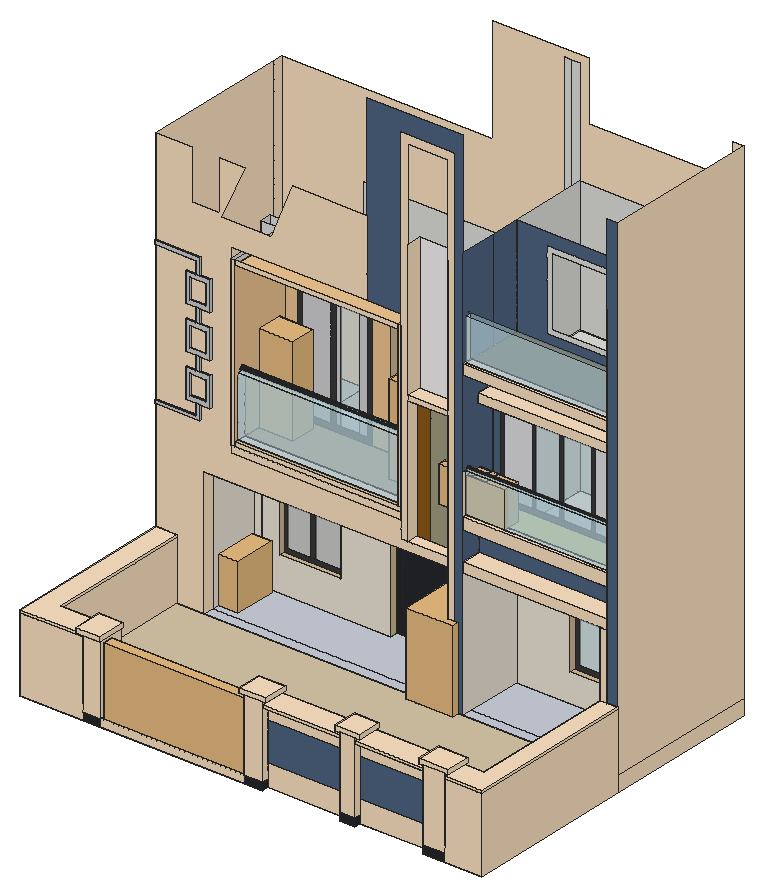
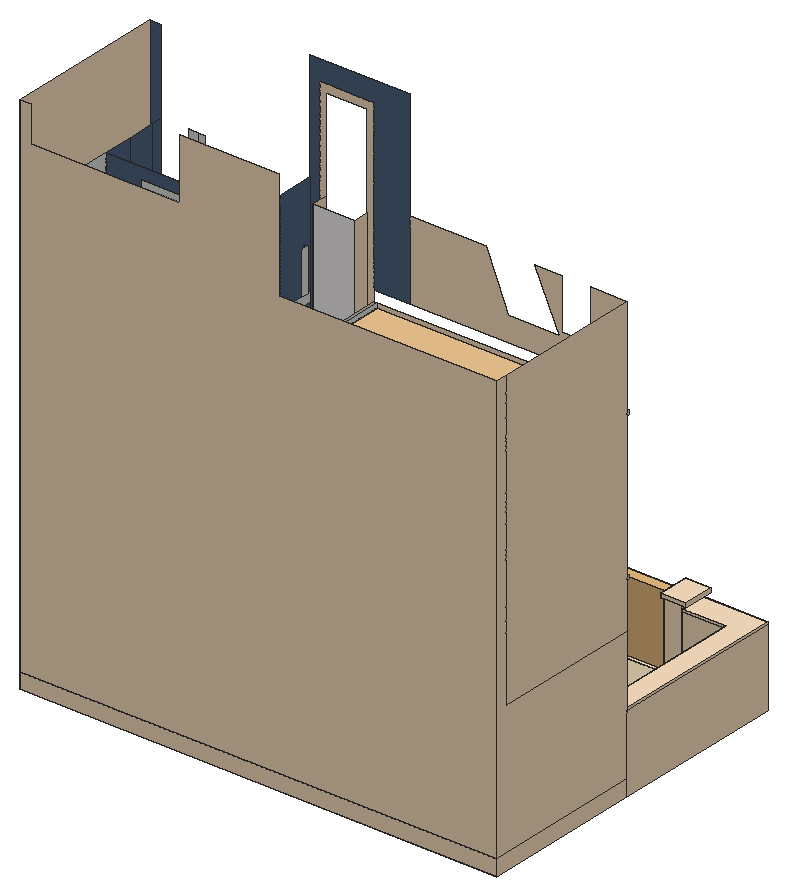
# SketchUp Ruby script. Lengths in inches.
U = 1.inch
M = Sketchup.active_model
def pt(a) = Geom::Point3d.new(a.map { |v| v * U })
def face(e, loops, mat)
  f = e.add_face(loops[0].map { |a| pt(a) })
  loops[1..].each { |l| e.add_face(l.map { |a| pt(a) }).erase! }
  f.material = f.back_material = mat if mat
  f
end
# faces: each face lists its corners as indices into pts; further lists are holes
def faces(e, pts, list, mat = nil) = list.each { |f| face(e, (f[0].is_a?(Array) ? f : [f]).map { |l| l.map { |i| pts[i] } }, mat) }
# xy, xz, yz: faces in a plane at the given z, y or x. An outline is a flat list of corners, or four numbers for a rectangle; further outlines are holes
def ring(l) = l.size == 4 ? [[l[0], l[1]], [l[2], l[1]], [l[2], l[3]], [l[0], l[3]]] : l.each_slice(2).to_a
def flat(e, list, mat, &to3) = list.each { |f| face(e, (f[0].is_a?(Array) ? f : [f]).map { |l| ring(l).map { |u, v| to3.(u, v) } }, mat) }
def xy(e, z, list, mat = nil) = flat(e, list, mat) { |x, y| [x, y, z] }
def xz(e, y, list, mat = nil) = flat(e, list, mat) { |x, z| [x, y, z] }
def yz(e, x, list, mat = nil) = flat(e, list, mat) { |y, z| [x, y, z] }
def lines(e, pts, list) = list.each { |a, b| e.add_line(pt(pts[a]), pt(pts[b])) }
# prism: a flat outline (further loops are holes) pulled along v
def prism(e, loops, v, mat = nil)
  f = face(e, loops, mat); d = Geom::Vector3d.new(v.map { |x| x * U })
  f.pushpull(f.normal.samedirection?(d) ? d.length : -d.length)
end
def box(e, o, s, mat = nil) = prism(e, [[o, [o[0] + s[0], o[1], o[2]], [o[0] + s[0], o[1] + s[1], o[2]], [o[0], o[1] + s[1], o[2]]]], [0, 0, s[2]], mat)
def at(x, y, z, deg = 0) = Geom::Transformation.translation(pt([x, y, z])) * Geom::Transformation.rotation(ORIGIN, Z_AXIS, deg.degrees)
def axes(o, x, y, z) = Geom::Transformation.new([*x, 0, *y, 0, *z, 0, *pt(o).to_a, 1])
def part(name) = M.definitions.add(name)
# library, detail: a bought-in or finely detailed component or shape, given as its bounding box
def library(name, o, s) = part(name).tap { |d| box(d.entities, o, s) }
def detail(e, o, s) = box(e.add_group.entities, o, s)
def put(e, d, t, mat = nil) = e.add_instance(d, t).tap { |i| i.material = mat if mat }
def group(e, t, mat = nil) = e.add_group.tap { |g| g.transformation = t; g.material = mat if mat }.entities
root = M.entities
M.materials.add("[0012_Bisque]").color = [255, 228, 196]
M.materials.add("[0036_BurlyWood]").color = [242, 200, 147]
M.materials.add("[Blinds Vertical Pattern]").color = [227, 227, 229]
M.materials.add("[Blinds Vertical Pattern]1").color = [212, 212, 214]
M.materials.add("[Blinds Weave]").color = [141, 91, 25]
M.materials.add("[Carpet Diamond Olive]").color = [87, 77, 61]
M.materials.add("[Carpet Diamond Yellow]").color = [226, 217, 124]
M.materials.add("[Carpet Pattern Leaf Squares Tan]").color = [181, 154, 125]
M.materials.add("[Carrera Marble]").color = [207, 207, 207]
M.materials.add("[Color M07]").color = [58, 58, 58]
M.materials.add("[Field Rectangle Tile]1").color = [239, 231, 218]
M.materials.add("[Field Square Tile]").color = [217, 201, 169]
M.materials.add("[Formica Beige]").color = [211, 187, 149]
M.materials.add("[Formica Graystone]").color = [149, 146, 135]
M.materials.add("[Formica Laminate Dark]").color = [38, 40, 45]
M.materials.add("[Formica Laminate Dark]1").color = [50, 53, 60]
M.materials.add("[Leather Blue]").color = [80, 102, 132]
M.materials.add("[Marble Carrara Floor Tile]").color = [204, 208, 219]
M.materials.add("[Stone Coursed Rough]").color = [165, 160, 130]
M.materials.add("[Stone Vein Gray]1").color = [247, 245, 245]
M.materials.add("[Translucent Glass Gray]").color = [188, 188, 188]
M.materials["[Translucent Glass Gray]"].alpha = 0.5
M.materials.add("[Translucent Glass Safety]").color = [204, 235, 244]
M.materials["[Translucent Glass Safety]"].alpha = 0.5
c1 = library("Gate_Lasercut_10ftx6ft_Kalil",[-0.15,-3.25,-0.15],[120,5.625,60.3])
c2 = library("Sem+nome",[-20.92,-6.25,0],[92.79,42.83,52.11])
c3 = library("chau cay",[-24.34,-109.24,0],[56.46,62.58,79.69])
xy(root,0,[[0,12.125,0,439.49,1160.87,439.49,1160.87,12.125,1013.97,12.125,1013.97,28.875,841.91,28.875,841.91,12.125,803.6875,12.125,803.6875,28.875,609.92,28.875,609.92,12.125],[0,439.49,1160.87,835.03]])
xy(root,20.125,[[202.63,12.125,561.64,73.77]],"[0012_Bisque]")
xy(root,38.625,[[0,439.49,0,835.03,1160.87,835.03,1160.87,439.49,1134.07,439.49,1134.07,808.22,138.99,808.22,138.99,597.14,120.87,597.14,120.87,439.49],[733.59,439.49,748.59,808.22],[748.59,439.49,771.27,808.22],[1117.13,439.49,1134.07,466.29],[1117.13,466.29,1134.07,607.94],
  [138.99,597.14,464.95,637.26],[685.01,597.14,733.59,637.26],[771.27,607.94,1134.07,637.26],[464.95,615.89,685.01,637.26],[138.99,637.26,733.59,808.22],
  [771.27,637.26,1134.07,808.22]])
xy(root,38.625,[[52.38,73.77,1117.13,439.49]],"[Field Square Tile]")
xy(root,38.625,[[120.87,439.49,733.59,466.29],[771.27,439.49,1117.13,466.29],[120.87,466.29,733.59,466.29,733.59,597.14,685.01,597.14,685.01,615.89,464.95,615.89,464.95,597.14,120.87,597.14],[771.27,466.29,1117.13,607.94]],"[Marble Carrara Floor Tile]")
xy(root,109.25,[[906.3,607.94,1097.3,624.38]],"[Formica Beige]")
xy(root,124.9,[[184.28,597.14,337.97,609.77]],"[Formica Beige]")
xy(root,186.76,[[0,12.125,0,439.49,52.38,439.49,52.38,73.77,158.51,73.77,158.51,12.125],[609.92,12.125,803.6875,28.875],[1067.46,12.125,1067.46,73.77,1117.13,73.77,1117.13,439.49,1160.87,439.49,1160.87,12.125],[609.92,28.875,803.6875,73.77],[841.91,28.875,1013.97,73.77]])
xy(root,186.76,[[841.91,12.125,1013.97,28.875]],"[0012_Bisque]")
xy(root,193.57,[[0,12.125,158.51,12.125,158.51,73.77,52.38,73.77,52.38,439.49,0,439.49],[609.92,12.125,803.6875,73.77],[841.91,12.125,1013.97,73.77],[1067.46,12.125,1160.87,12.125,1160.87,439.49,1117.13,439.49,1117.13,73.77,1067.46,73.77]],"[0012_Bisque]")
xy(root,199.3125,[[158.51,12.125,202.63,73.77],[561.64,12.125,609.92,73.77],[609.92,12.125,617.61,73.77],[791.875,12.125,803.6875,73.77],[803.6875,12.125,841.91,73.77],
  [841.91,12.125,853.91,73.77],[1003.78,12.125,1013.97,73.77],[1013.97,12.125,1067.46,73.77],[1067.46,12.125,1076.52,73.77]])
xy(root,199.3125,[[148.76,0,202.63,12.125],[202.63,0,209.69,73.77],[148.76,12.125,158.51,73.77],[551.08,12.125,561.64,73.77]],"[0012_Bisque]")
xy(root,210.75,[[148.76,0,209.69,73.77],[551.08,12.125,617.61,73.77],[791.875,12.125,853.91,73.77],[1003.78,12.125,1076.52,73.77]],"[0012_Bisque]")
xy(root,316.75,[[906.3,607.94,1097.3,624.38]],"[Formica Beige]")
xy(root,323.25,[[464.95,615.89,685.01,637.26]])
xy(root,323.25,[[464.95,597.14,685.01,615.89]],"[Formica Beige]")
xy(root,325.09,[[184.28,597.14,337.97,609.77]],"[Formica Beige]")
xy(root,359.3125,[[1117.13,439.49,1134.07,466.29],[1117.13,466.29,1134.07,607.94],[0,597.14,138.99,637.26],[138.99,597.14,733.59,637.26],[771.27,607.94,1134.07,637.26],
  [0,637.26,138.99,808.22],[138.99,637.26,733.59,808.22],[771.27,637.26,1134.07,808.22]])
xy(root,359.3125,[[120.87,439.49,733.59,597.14],[771.27,439.49,1117.13,607.94]],"[0036_BurlyWood]")
xy(root,381.625,[[633.21,439.49,733.59,468.8]],"[0012_Bisque]")
xy(root,383.3125,[[771.27,490.72,1134.07,808.22]])
xy(root,383.3125,[[771.27,439.49,1134.07,490.72]],"[0012_Bisque]")
xy(root,442.75,[[187.18,439.49,197.99,595.47],[197.99,439.49,615.34,595.47]])
xy(root,453.1875,[[607.9,439.49,615.34,595.47],[197.99,449.39,607.9,470.4375]])
xy(root,453.1875,[[197.99,470.4375,607.9,595.47]],"[Carpet Pattern Leaf Squares Tan]")
xy(root,453.1875,[[197.99,439.49,607.9,449.39],[466.17,595.47,560.67,614.72]],"[Formica Beige]")
xy(root,455.55,[[771.27,439.49,1134.07,490.72],[771.27,490.72,1134.07,532.66]])
xy(root,472.81,[[0,434.86,112.84,439.49]],"[Carrera Marble]")
xy(root,480.87,[[0,434.86,104.75,439.49]],"[Carrera Marble]")
xy(root,486.24,[[771.27,448.11,1134.07,459.625]])
xy(root,486.24,[[771.27,439.49,1134.07,448.11]],"[0012_Bisque]")
xy(root,486.24,[[771.27,459.625,1134.07,532.66]],"[Carpet Diamond Yellow]")
xy(root,509.49,[[104.75,434.86,112.84,439.49]])
xy(root,509.49,[[77.56,434.86,104.75,439.49],[112.84,434.86,139.68,439.49]],"[Carrera Marble]")
xy(root,520.32,[[88.38,434.86,128.86,439.49]],"[Carrera Marble]")
xy(root,571.79,[[88.38,434.86,128.86,439.49]],"[Carrera Marble]")
xy(root,582.62,[[104.75,434.86,112.84,439.49]])
xy(root,582.62,[[77.56,434.86,104.75,439.49],[112.84,434.86,139.68,439.49]],"[Carrera Marble]")
xy(root,586.49,[[771.27,448.11,1134.07,459.625]],"[Translucent Glass Safety]")
xy(root,604.3125,[[197.99,449.39,607.9,470.4375]],"[Translucent Glass Safety]")
xy(root,617.49,[[104.75,434.86,112.84,439.49]])
xy(root,617.49,[[77.56,434.86,104.75,439.49],[112.84,434.86,139.68,439.49]],"[Carrera Marble]")
xy(root,628.32,[[88.38,434.86,128.86,439.49]],"[Carrera Marble]")
xy(root,679.79,[[88.38,434.86,128.86,439.49]],"[Carrera Marble]")
xy(root,690.62,[[104.75,434.86,112.84,439.49]])
xy(root,690.62,[[77.56,434.86,104.75,439.49],[112.84,434.86,139.68,439.49]],"[Carrera Marble]")
xy(root,699.47,[[633.21,439.49,733.59,468.8]],"[0012_Bisque]")
xy(root,711.375,[[633.21,439.49,733.59,477.49]],"[0012_Bisque]")
xy(root,722.1,[[771.27,487.6,1134.07,532.66]],"[Leather Blue]")
xy(root,725.99,[[77.56,434.86,104.75,439.49],[104.75,434.86,112.84,439.49],[112.84,434.86,139.68,439.49]])
xy(root,736.82,[[88.38,434.86,128.86,439.49]],"[Carrera Marble]")
xy(root,744.1875,[[771.27,532.66,1134.07,808.22]])
xy(root,744.1875,[[771.27,487.6,1134.07,532.66]],"[0012_Bisque]")
xy(root,788.29,[[88.38,434.86,128.86,439.49]],"[Carrera Marble]")
xy(root,799.12,[[104.75,434.86,112.84,439.49]])
xy(root,799.12,[[77.56,434.86,104.75,439.49],[112.84,434.86,139.68,439.49]],"[Carrera Marble]")
xy(root,805.03,[[466.17,595.47,560.67,614.72]],"[Formica Beige]")
xy(root,805.4,[[771.27,532.66,1134.07,607.94]])
xy(root,805.4,[[771.27,439.49,1134.07,532.66]],"[0012_Bisque]")
xy(root,829.28,[[771.27,448.03,1134.07,465.29]])
xy(root,829.28,[[771.27,439.49,1134.07,448.03]],"[0012_Bisque]")
xy(root,829.28,[[771.27,465.29,1134.07,607.94]],"[Carpet Diamond Olive]")
xy(root,831.0625,[[0,434.86,104.75,439.49]],"[Carrera Marble]")
xy(root,840.93,[[0,434.86,112.84,439.49]],"[Carrera Marble]")
xy(root,851.9375,[[197.99,439.49,607.9,595.47]],"[0036_BurlyWood]")
xz(root,0,[[148.76,199.3125,209.69,210.75]],"[0012_Bisque]")
xz(root,12.125,[[0,0,158.51,186.76],[202.63,0,561.64,20.125],[1067.46,0,1160.87,186.76],[158.51,19.3125,202.63,199.3125],[561.64,19.3125,609.92,199.3125],
  [803.6875,19.3125,841.91,199.3125],[1013.97,19.3125,1067.46,199.3125],[0,186.76,158.51,193.57],[609.92,186.76,803.6875,193.57],[841.91,186.76,1013.97,193.57],
  [1067.46,186.76,1160.87,193.57],[551.08,199.3125,617.61,210.75],[791.875,199.3125,853.91,210.75],[1003.78,199.3125,1076.52,210.75]],"[0012_Bisque]")
xz(root,12.125,[[158.51,0,202.63,19.3125],[561.64,0,609.92,19.3125],[803.6875,0,841.91,19.3125],[1013.97,0,1067.46,19.3125]],"[Formica Laminate Dark]")
xz(root,28.875,[[609.92,0,803.6875,55.35],[841.91,0,1013.97,55.35],[609.92,152.16,803.6875,186.76],[841.91,152.16,1013.97,186.76]],"[0012_Bisque]")
xz(root,28.875,[[609.92,55.35,803.6875,152.16],[841.91,55.35,1013.97,152.16]],"[Leather Blue]")
xz(root,73.77,[[202.63,20.125,561.64,38.625],[52.38,38.625,158.51,186.76],[158.51,38.625,202.63,199.3125],[561.64,38.625,609.92,199.3125],[609.92,38.625,803.6875,186.76],
  [803.6875,38.625,841.91,199.3125],[841.91,38.625,1013.97,186.76],[1013.97,38.625,1067.46,199.3125],[1067.46,38.625,1117.13,186.76],[52.38,186.76,158.51,193.57],
  [609.92,186.76,803.6875,193.57],[841.91,186.76,1013.97,193.57],[1067.46,186.76,1117.13,193.57],[148.76,199.3125,209.69,210.75],[551.08,199.3125,617.61,210.75],
  [791.875,199.3125,853.91,210.75],[1003.78,199.3125,1076.52,210.75]],"[0012_Bisque]")
xz(root,434.86,[[0,472.81,112.84,472.81,112.84,509.49,104.75,509.49,104.75,480.87,0,480.87],[[77.56,509.49,139.68,582.62],[88.38,520.32,128.86,571.79]],[104.75,582.62,112.84,617.49],[[77.56,617.49,139.68,690.62],[88.38,628.32,128.86,679.79]],[104.75,690.62,112.84,725.99],
  [[77.56,725.99,139.68,799.12],[88.38,736.82,128.86,788.29]],[104.75,799.12,112.84,799.12,112.84,840.93,0,840.93,0,831.0625,104.75,831.0625]],"[Carrera Marble]")
xz(root,439.49,[[0,0,1160.87,38.625],[0,38.625,52.38,186.76],[1117.13,38.625,1134.07,186.76],[1134.07,38.625,1160.87,186.76],[0,186.76,52.38,193.57],
  [1117.13,186.76,1134.07,193.57],[1134.07,186.76,1160.87,193.57],[0,472.81,0,480.87,104.75,480.87,104.75,509.49,112.84,509.49,112.84,472.81],[[77.56,509.49,139.68,582.62],[88.38,520.32,128.86,571.79]],[104.75,582.62,112.84,617.49],
  [[77.56,617.49,139.68,690.62],[88.38,628.32,128.86,679.79]],[104.75,690.62,112.84,725.99],[[77.56,725.99,139.68,799.12],[88.38,736.82,128.86,788.29]],[104.75,799.12,104.75,831.0625,0,831.0625,0,840.93,112.84,840.93,112.84,799.12]])
xz(root,439.49,[[52.38,38.625,120.87,38.625,120.87,359.3125,733.59,359.3125,733.59,381.625,615.34,381.625,615.34,424.875,187.18,424.875,187.18,889,529.97,889,529.97,1079.8125,342.79,1079.8125,298.76,967.96,290.72,947.54,162.87,947.54,172.3,967.96,223.93,1079.8125,159.99,1079.8125,159.99,956.62,89.49,956.62,89.49,1079.8125,0,1079.8125,0,840.93,112.84,840.93,112.84,799.12,139.68,799.12,139.68,725.99,112.84,725.99,112.84,690.62,139.68,690.62,139.68,617.49,112.84,617.49,112.84,582.62,139.68,582.62,139.68,509.49,112.84,509.49,112.84,472.81,0,472.81,0,193.57,52.38,193.57],[733.59,38.625,748.59,38.625,748.59,1297.21,615.34,1297.21,615.34,381.625,633.21,381.625,633.21,1276.62,733.59,1276.62],[1117.13,193.57,1134.07,359.3125],[771.27,359.3125,1134.07,383.3125],[187.18,424.875,615.34,442.75],
  [187.18,442.75,197.99,862.4375],[197.99,442.75,615.34,453.1875],[607.9,453.1875,615.34,862.4375],[771.27,455.55,1134.07,486.24],[0,480.87,104.75,480.87,104.75,509.49,77.56,509.49,77.56,582.62,104.75,582.62,104.75,617.49,77.56,617.49,77.56,690.62,104.75,690.62,104.75,725.99,77.56,725.99,77.56,799.12,104.75,799.12,104.75,831.0625,0,831.0625],
  [88.38,520.32,128.86,571.79],[88.38,628.32,128.86,679.79],[633.21,699.47,733.59,711.375],[88.38,736.82,128.86,788.29],[771.27,805.4,1134.07,829.28],
  [197.99,851.9375,607.9,862.4375]],"[0012_Bisque]")
xz(root,439.49,[[748.59,38.625,771.27,38.625,771.27,1345.9375,529.97,1345.9375,529.97,889,615.34,889,615.34,1297.21,748.59,1297.21],[1134.07,193.57,1160.87,1284.8125]],"[Leather Blue]")
xz(root,448.03,[[771.27,829.28,1134.07,933.85]],"[Translucent Glass Safety]")
xz(root,448.11,[[771.27,486.24,1134.07,586.49]],"[Translucent Glass Safety]")
xz(root,449.39,[[197.99,453.1875,607.9,604.3125]],"[Translucent Glass Safety]")
xz(root,459.625,[[771.27,486.24,1134.07,586.49]],"[Translucent Glass Safety]")
xz(root,465.29,[[771.27,829.28,1134.07,933.85]],"[Translucent Glass Safety]")
xz(root,466.29,[[1117.13,38.625,1134.07,359.3125]])
xz(root,468.8,[[633.21,381.625,666.82,699.47]],"[Blinds Weave]")
xz(root,468.8,[[666.82,381.625,733.59,699.47]],"[Stone Coursed Rough]")
xz(root,470.4375,[[197.99,453.1875,607.9,604.3125]],"[Translucent Glass Safety]")
xz(root,477.49,[[633.21,711.375,733.59,1050.61]],"[Stone Vein Gray]1")
xz(root,487.6,[[771.27,722.1,1134.07,744.1875]],"[0012_Bisque]")
xz(root,490.72,[[771.27,383.3125,1134.07,455.55]],"[Leather Blue]")
xz(root,532.66,[[771.27,455.55,1134.07,486.24]])
xz(root,532.66,[[802.74,499.05,871.07,697.27],[1031.83,499.05,1096.89,697.27]],"[Blinds Vertical Pattern]")
xz(root,532.66,[[[789.93,486.24,1109.69,710.08],[802.74,499.05,1096.89,697.27]],[871.07,499.05,880.26,697.27],[942.07,499.05,951.26,697.27],[1022.63,499.05,1031.83,697.27]],"[Color M07]")
xz(root,532.66,[[771.27,486.24,789.93,486.24,789.93,710.08,1109.69,710.08,1109.69,486.24,1134.07,486.24,1134.07,722.1,771.27,722.1],[771.27,744.1875,1134.07,805.4]],"[Leather Blue]")
xz(root,532.66,[[880.26,499.05,942.07,697.27],[951.26,499.05,1022.63,697.27]],"[Translucent Glass Safety]")
xz(root,595.47,[[138.99,423.9375,187.18,862.4375],[187.18,423.9375,615.34,442.75],[187.18,442.75,197.99,862.4375],[197.99,442.75,615.34,453.1875],[607.9,453.1875,615.34,862.4375],
  [197.99,851.9375,228.43,862.4375],[228.43,851.9375,607.9,862.4375]])
xz(root,595.47,[[197.99,453.1875,229.59,453.1875,229.59,794.8125,420.59,794.8125,420.59,453.1875,466.17,453.1875,466.17,805.03,560.67,805.03,560.67,453.1875,607.9,453.1875,607.9,851.9375,197.99,851.9375]],"[0036_BurlyWood]")
xz(root,595.47,[[244.92,468.52,314.64,779.48],[326.8,468.52,339.12,779.48],[387.01,468.52,405.25,779.48]],"[Blinds Vertical Pattern]1")
xz(root,595.47,[[[229.59,453.1875,420.59,794.8125],[244.92,468.52,405.25,779.48]],[314.64,468.52,326.8,779.48]],"[Color M07]")
xz(root,595.47,[[339.12,468.52,387.01,779.48]],"[Translucent Glass Safety]")
xz(root,597.14,[[120.87,38.625,138.99,359.3125],[[138.99,38.625,464.95,38.625,464.95,323.25,685.01,323.25,685.01,38.625,733.59,38.625,733.59,359.3125,138.99,359.3125],[184.28,124.9,337.97,325.09]]],"[Field Rectangle Tile]1")
xz(root,607.94,[[1117.13,38.625,1134.07,359.3125],[771.27,805.4,1134.07,829.28],[[846.73,850.66,1046.48,1050.41],[860.01,863.95,1033.1875,1037.12]]])
xz(root,607.94,[[[771.27,38.625,1117.13,359.3125],[906.3,109.25,1097.3,316.75]]],"[Field Rectangle Tile]1")
xz(root,607.94,[[[771.27,829.28,1134.07,1079.8125],[846.73,850.66,1046.48,1050.41]]],"[Leather Blue]")
xz(root,609.77,[[[184.28,124.9,337.97,325.09],[195.12,135.74,327.13,314.26]],[253.15,135.74,266.31,314.26]],"[Color M07]")
xz(root,609.77,[[195.12,135.74,253.15,314.26],[266.31,135.74,327.13,314.26]],"[Translucent Glass Gray]")
xz(root,614.72,[[466.17,453.1875,560.67,805.03]],"[Formica Laminate Dark]1")
xz(root,615.89,[[[464.95,38.625,685.01,323.25],[480.3,53.97,669.67,307.91]],[480.3,53.97,669.67,307.91]],"[Formica Laminate Dark]")
xz(root,623.86,[[138.99,423.9375,228.43,862.4375]])
xz(root,624.38,[[[906.3,109.25,1097.3,316.75],[917.25,120.2,1086.35,305.79]],[993.57,120.2,1003.36,305.79]],"[Color M07]")
xz(root,624.38,[[917.25,120.2,993.57,305.79],[1003.36,120.2,1086.35,305.79]],"[Translucent Glass Safety]")
xz(root,637.26,[[138.99,38.625,138.99,359.3125,733.59,359.3125,733.59,38.625,685.01,38.625,685.01,323.25,464.95,323.25,464.95,38.625],[771.27,38.625,1134.07,359.3125]])
xz(root,808.22,[[138.99,38.625,733.59,359.3125],[733.59,38.625,748.59,1345.9375],[748.59,38.625,771.27,1345.9375],[771.27,38.625,1134.07,359.3125],[138.99,359.3125,733.59,423.9375],
  [771.27,359.3125,1134.07,383.3125],[771.27,383.3125,1134.07,744.1875],[228.43,423.9375,733.59,889],[771.27,744.1875,1134.07,1079.8125]])
xz(root,835.03,[[0,0,1160.87,38.625],[0,38.625,0,1079.8125,529.97,1079.8125,529.97,1345.9375,771.27,1345.9375,771.27,1197.6875,1134.07,1197.6875,1134.07,1284.8125,1160.87,1284.8125,1160.87,38.625]],"[0012_Bisque]")
yz(root,0,[[434.86,831.0625,439.49,840.93]])
yz(root,0,[[12.125,0,439.49,186.76],[439.49,0,835.03,38.625],[439.49,38.625,439.49,359.3125,808.22,359.3125,808.22,1079.8125,835.03,1079.8125,835.03,38.625],[12.125,186.76,439.49,193.57],[439.49,359.3125,808.22,1079.8125]],"[0012_Bisque]")
yz(root,0,[[434.86,472.81,439.49,480.87]],"[Carrera Marble]")
yz(root,52.38,[[73.77,38.625,439.49,186.76],[73.77,186.76,439.49,193.57]],"[0012_Bisque]")
yz(root,77.56,[[434.86,509.49,439.49,582.62],[434.86,617.49,439.49,690.62],[434.86,725.99,439.49,799.12]],"[Carrera Marble]")
yz(root,88.38,[[434.86,520.32,439.49,571.79],[434.86,628.32,439.49,679.79],[434.86,736.82,439.49,788.29]],"[Carrera Marble]")
yz(root,104.75,[[434.86,480.87,439.49,509.49],[434.86,582.62,439.49,617.49],[434.86,690.62,439.49,725.99],[434.86,799.12,439.49,831.0625]],"[Carrera Marble]")
yz(root,112.84,[[434.86,472.81,439.49,509.49],[434.86,582.62,439.49,617.49],[434.86,690.62,439.49,725.99],[434.86,799.12,439.49,840.93]],"[Carrera Marble]")
yz(root,120.87,[[439.49,38.625,466.29,359.3125]],"[0012_Bisque]")
yz(root,120.87,[[466.29,38.625,597.14,359.3125]],"[Field Rectangle Tile]1")
yz(root,128.86,[[434.86,520.32,439.49,571.79],[434.86,628.32,439.49,679.79],[434.86,736.82,439.49,788.29]],"[Carrera Marble]")
yz(root,138.99,[[597.14,38.625,637.26,359.3125],[637.26,38.625,808.22,359.3125],[595.47,423.9375,623.86,862.4375]])
yz(root,139.68,[[434.86,509.49,439.49,582.62],[434.86,617.49,439.49,690.62],[434.86,725.99,439.49,799.12]],"[Carrera Marble]")
yz(root,148.76,[[0,199.3125,73.77,210.75]],"[0012_Bisque]")
yz(root,158.51,[[12.125,38.625,73.77,186.76],[12.125,186.76,73.77,193.57]])
yz(root,158.51,[[12.125,193.57,73.77,199.3125]],"[0012_Bisque]")
yz(root,184.28,[[597.14,124.9,609.77,325.09]],"[Formica Beige]")
yz(root,187.18,[[439.49,442.75,595.47,862.4375]])
yz(root,197.99,[[439.49,442.75,595.47,453.1875],[449.39,453.1875,470.4375,604.3125],[439.49,851.9375,595.47,862.4375]])
yz(root,197.99,[[[439.49,453.1875,449.39,453.1875,449.39,604.3125,470.4375,604.3125,470.4375,453.1875,595.47,453.1875,595.47,851.9375,439.49,851.9375],[459.35,608.19,458.02,608.37,456.79,608.88,455.73,609.69,454.91,610.76,454.4,611.99,454.22,613.32,454.4,614.65,454.91,615.88,455.73,616.94,456.79,617.76,458.02,618.27,459.35,618.44,460.68,618.27,461.91,617.76,462.97,616.94,463.79,615.88,464.3,614.65,464.47,613.32,464.3,611.99,463.79,610.76,462.97,609.69,461.91,608.88,460.68,608.37]]],"[0036_BurlyWood]")
yz(root,202.63,[[12.125,20.125,73.77,199.3125]],"[0012_Bisque]")
yz(root,209.69,[[0,199.3125,73.77,210.75]],"[0012_Bisque]")
yz(root,337.97,[[597.14,124.9,609.77,325.09]],"[Formica Beige]")
yz(root,464.95,[[615.89,38.625,637.26,323.25]])
yz(root,464.95,[[597.14,38.625,615.89,323.25]],"[Formica Beige]")
yz(root,466.17,[[595.47,453.1875,614.72,805.03]],"[Formica Beige]")
yz(root,551.08,[[12.125,199.3125,73.77,210.75]],"[0012_Bisque]")
yz(root,560.67,[[595.47,453.1875,614.72,805.03]],"[Formica Beige]")
yz(root,561.64,[[12.125,20.125,73.77,199.3125]],"[0012_Bisque]")
yz(root,607.9,[[449.39,453.1875,470.4375,604.3125],[459.35,608.19,460.68,608.37,461.91,608.88,462.97,609.69,463.79,610.76,464.3,611.99,464.47,613.32,464.3,614.65,463.79,615.88,462.97,616.94,461.91,617.76,460.68,618.27,459.35,618.44,458.02,618.27,456.79,617.76,455.73,616.94,454.91,615.88,454.4,614.65,454.22,613.32,454.4,611.99,454.91,610.76,455.73,609.69,456.79,608.88,458.02,608.37],[439.49,851.9375,595.47,862.4375]])
yz(root,607.9,[[[439.49,453.1875,439.49,851.9375,595.47,851.9375,595.47,453.1875,470.4375,453.1875,470.4375,604.3125,449.39,604.3125,449.39,453.1875],[459.35,608.19,460.68,608.37,461.91,608.88,462.97,609.69,463.79,610.76,464.3,611.99,464.47,613.32,464.3,614.65,463.79,615.88,462.97,616.94,461.91,617.76,460.68,618.27,459.35,618.44,458.02,618.27,456.79,617.76,455.73,616.94,454.91,615.88,454.4,614.65,454.22,613.32,454.4,611.99,454.91,610.76,455.73,609.69,456.79,608.88,458.02,608.37]]],"[0036_BurlyWood]")
yz(root,609.92,[[28.875,38.625,73.77,186.76],[12.125,186.76,73.77,193.57]])
yz(root,609.92,[[12.125,19.3125,28.875,186.76],[12.125,193.57,73.77,199.3125]],"[0012_Bisque]")
yz(root,609.92,[[12.125,0,28.875,19.3125]],"[Formica Laminate Dark]")
yz(root,615.34,[[439.49,423.9375,595.47,442.75],[439.49,442.75,595.47,453.1875],[439.49,453.1875,595.47,862.4375]])
yz(root,617.61,[[12.125,199.3125,73.77,210.75]],"[0012_Bisque]")
yz(root,633.21,[[439.49,381.625,468.8,699.47],[439.49,711.375,477.49,1050.61]],"[0012_Bisque]")
yz(root,685.01,[[615.89,38.625,637.26,323.25]])
yz(root,685.01,[[597.14,38.625,615.89,323.25]],"[Formica Beige]")
yz(root,733.59,[[597.14,38.625,637.26,359.3125],[637.26,38.625,808.22,359.3125],[439.49,359.3125,466.29,381.625],[466.29,359.3125,597.14,359.3125,597.14,423.9375,468.8,423.9375,468.8,381.625,466.29,381.625],[597.14,359.3125,637.26,423.9375],
  [637.26,359.3125,808.22,423.9375],[595.47,423.9375,597.14,889],[597.14,423.9375,623.86,889],[623.86,423.9375,637.26,889],[637.26,423.9375,808.22,889]])
yz(root,733.59,[[439.49,381.625,466.29,423.9375],[466.29,381.625,468.8,423.9375],[439.49,423.9375,468.8,699.47],[439.49,711.375,477.49,1050.61]],"[0012_Bisque]")
yz(root,733.59,[[439.49,38.625,597.14,359.3125]],"[Field Rectangle Tile]1")
yz(root,771.27,[[607.94,38.625,637.26,359.3125],[637.26,38.625,808.22,359.3125],[439.49,359.3125,607.94,383.3125],[607.94,359.3125,637.26,383.3125],[637.26,359.3125,808.22,383.3125],
  [490.72,383.3125,607.94,383.3125,607.94,744.1875,487.6,744.1875,487.6,722.1,532.66,722.1,532.66,455.55,490.72,455.55],[607.94,383.3125,637.26,744.1875],[637.26,383.3125,808.22,744.1875],[439.49,455.55,532.66,486.24],[448.11,486.24,459.625,586.49],
  [532.66,744.1875,808.22,744.1875,808.22,1079.8125,607.94,1079.8125,607.94,805.4,532.66,805.4],[439.49,805.4,532.66,829.28],[532.66,805.4,607.94,829.28],[448.03,829.28,465.29,933.85]])
yz(root,771.27,[[439.49,486.24,448.11,586.49]],"[0012_Bisque]")
yz(root,771.27,[[439.49,38.625,607.94,359.3125]],"[Field Rectangle Tile]1")
yz(root,771.27,[[439.49,383.3125,490.72,455.55],[[459.625,486.24,532.66,486.24,532.66,722.1,487.6,722.1,487.6,744.1875,532.66,744.1875,532.66,805.4,439.49,805.4,439.49,586.49,459.625,586.49],[453.26,588.64,452.41,588.75,451.63,589.07,450.95,589.59,450.4375,590.26,450.11,591.04,450,591.88,450.11,592.72,450.43,593.51,450.94,594.18,451.61,594.7,452.4,595.03,453.24,595.14,454.08,595.03,454.86,594.71,455.54,594.19,456.06,593.52,456.38,592.74,456.5,591.9,456.39,591.06,456.07,590.27,455.55,589.6,454.88,589.08,454.1,588.75]],[[439.49,829.28,448.03,829.28,448.03,933.85,465.29,933.85,465.29,829.28,532.66,829.28,532.66,1079.8125,439.49,1079.8125],[458.49,936.6,457.68,936.71,456.93,937.02,456.28,937.51,455.78,938.16,455.47,938.92,455.36,939.72,455.47,940.53,455.78,941.29,456.28,941.93,456.93,942.43,457.68,942.74,458.49,942.85,459.3,942.74,460.05,942.43,460.7,941.93,461.19,941.29,461.51,940.53,461.61,939.72,461.51,938.92,461.19,938.16,460.7,937.51,460.05,937.02,459.3,936.71]],[532.66,829.28,607.94,1079.8125]],"[Leather Blue]")
yz(root,791.875,[[12.125,199.3125,73.77,210.75]],"[0012_Bisque]")
yz(root,803.6875,[[12.125,186.76,73.77,193.57]])
yz(root,803.6875,[[12.125,19.3125,28.875,186.76],[12.125,193.57,73.77,199.3125]],"[0012_Bisque]")
yz(root,803.6875,[[12.125,0,28.875,19.3125]],"[Formica Laminate Dark]")
yz(root,841.91,[[28.875,38.625,73.77,186.76],[12.125,186.76,73.77,193.57]])
yz(root,841.91,[[12.125,19.3125,28.875,186.76],[12.125,193.57,73.77,199.3125]],"[0012_Bisque]")
yz(root,841.91,[[12.125,0,28.875,19.3125]],"[Formica Laminate Dark]")
yz(root,853.91,[[12.125,199.3125,73.77,210.75]],"[0012_Bisque]")
yz(root,906.3,[[607.94,109.25,624.38,316.75]],"[Formica Beige]")
yz(root,1003.78,[[12.125,199.3125,73.77,210.75]],"[0012_Bisque]")
yz(root,1013.97,[[28.875,38.625,73.77,186.76],[12.125,186.76,73.77,193.57]])
yz(root,1013.97,[[12.125,19.3125,28.875,38.625],[12.125,38.625,28.875,186.76],[12.125,193.57,73.77,199.3125]],"[0012_Bisque]")
yz(root,1013.97,[[12.125,0,28.875,19.3125]],"[Formica Laminate Dark]")
yz(root,1067.46,[[12.125,38.625,73.77,186.76],[12.125,186.76,73.77,193.57]])
yz(root,1067.46,[[12.125,193.57,73.77,199.3125]],"[0012_Bisque]")
yz(root,1076.52,[[12.125,199.3125,73.77,210.75]],"[0012_Bisque]")
yz(root,1097.3,[[607.94,109.25,624.38,316.75]],"[Formica Beige]")
yz(root,1117.13,[[73.77,38.625,439.49,186.76],[439.49,38.625,466.29,359.3125],[73.77,186.76,439.49,193.57]],"[0012_Bisque]")
yz(root,1117.13,[[466.29,38.625,607.94,359.3125]],"[Field Rectangle Tile]1")
yz(root,1134.07,[[439.49,38.625,466.29,359.3125],[466.29,38.625,607.94,359.3125],[607.94,38.625,637.26,359.3125],[637.26,38.625,808.22,359.3125],[439.49,359.3125,466.29,383.3125],
  [466.29,359.3125,607.94,383.3125],[607.94,359.3125,637.26,383.3125],[637.26,359.3125,808.22,383.3125],[490.72,383.3125,490.72,455.55,532.66,455.55,532.66,722.1,487.6,722.1,487.6,744.1875,607.94,744.1875,607.94,383.3125],[607.94,383.3125,637.26,744.1875],
  [637.26,383.3125,808.22,744.1875],[439.49,455.55,466.29,486.24],[466.29,455.55,532.66,486.24],[448.11,486.24,459.625,586.49],[453.26,588.64,454.1,588.75,454.88,589.08,455.55,589.6,456.07,590.27,456.39,591.06,456.5,591.9,456.38,592.74,456.06,593.52,455.54,594.19,454.86,594.71,454.08,595.03,453.24,595.14,452.4,595.03,451.61,594.7,450.94,594.18,450.43,593.51,450.11,592.72,450,591.88,450.11,591.04,450.4375,590.26,450.95,589.59,451.63,589.07,452.41,588.75],
  [532.66,744.1875,532.66,805.4,607.94,805.4,607.94,1079.8125,808.22,1079.8125,808.22,744.1875],[439.49,805.4,466.29,829.28],[466.29,805.4,532.66,829.28],[532.66,805.4,607.94,829.28],[448.03,829.28,465.29,933.85]])
yz(root,1134.07,[[439.49,486.24,448.11,586.49]],"[0012_Bisque]")
yz(root,1134.07,[[439.49,383.3125,466.29,455.55],[466.29,383.3125,490.72,455.55],[[459.625,486.24,459.625,586.49,439.49,586.49,439.49,805.4,466.29,805.4,466.29,486.24],[453.26,588.64,454.1,588.75,454.88,589.08,455.55,589.6,456.07,590.27,456.39,591.06,456.5,591.9,456.38,592.74,456.06,593.52,455.54,594.19,454.86,594.71,454.08,595.03,453.24,595.14,452.4,595.03,451.61,594.7,450.94,594.18,450.43,593.51,450.11,592.72,450,591.88,450.11,591.04,450.4375,590.26,450.95,589.59,451.63,589.07,452.41,588.75]],[466.29,486.24,466.29,805.4,532.66,805.4,532.66,744.1875,487.6,744.1875,487.6,722.1,532.66,722.1,532.66,486.24],[[439.49,829.28,439.49,1079.8125,466.29,1079.8125,466.29,829.28,465.29,829.28,465.29,933.85,448.03,933.85,448.03,829.28],[458.49,936.6,459.3,936.71,460.05,937.02,460.7,937.51,461.19,938.16,461.51,938.92,461.61,939.72,461.51,940.53,461.19,941.29,460.7,941.93,460.05,942.43,459.3,942.74,458.49,942.85,457.68,942.74,456.93,942.43,456.28,941.93,455.78,941.29,455.47,940.53,455.36,939.72,455.47,938.92,455.78,938.16,456.28,937.51,456.93,937.02,457.68,936.71]],
  [466.29,829.28,532.66,1079.8125],[532.66,829.28,607.94,1079.8125]],"[Leather Blue]")
yz(root,1160.87,[[12.125,0,439.49,186.76],[439.49,0,835.03,38.625],[439.49,38.625,835.03,1284.8125],[12.125,186.76,439.49,193.57]],"[0012_Bisque]")
p = [[1134.07,453.26,588.64],[1134.07,452.41,588.75],[771.27,452.41,588.75],[771.27,453.26,588.64],[1134.07,454.1,588.75],[771.27,454.1,588.75],
  [1134.07,451.63,589.07],[771.27,451.63,589.07],[1134.07,454.88,589.08],[771.27,454.88,589.08],[1134.07,450.95,589.59],[771.27,450.95,589.59],
  [1134.07,455.55,589.6],[771.27,455.55,589.6],[1134.07,450.4375,590.26],[771.27,450.4375,590.26],[1134.07,456.07,590.27],[771.27,456.07,590.27],
  [1134.07,450.11,591.04],[771.27,450.11,591.04],[1134.07,456.39,591.06],[771.27,456.39,591.06],[1134.07,450,591.88],[771.27,450,591.88],
  [1134.07,456.5,591.9],[771.27,456.5,591.9],[1134.07,450.11,592.72],[771.27,450.11,592.72],[1134.07,456.38,592.74],[771.27,456.38,592.74],
  [1134.07,450.43,593.51],[771.27,450.43,593.51],[1134.07,456.06,593.52],[771.27,456.06,593.52],[1134.07,450.94,594.18],[771.27,450.94,594.18],
  [1134.07,455.54,594.19],[771.27,455.54,594.19],[1134.07,451.61,594.7],[771.27,451.61,594.7],[1134.07,454.86,594.71],[771.27,454.86,594.71],
  [1134.07,452.4,595.03],[771.27,452.4,595.03],[1134.07,454.08,595.03],[771.27,454.08,595.03],[1134.07,453.24,595.14],[771.27,453.24,595.14],
  [607.9,459.35,608.19],[607.9,458.02,608.37],[197.99,458.02,608.37],[197.99,459.35,608.19],[607.9,460.68,608.37],[197.99,460.68,608.37],
  [607.9,456.79,608.88],[197.99,456.79,608.88],[607.9,461.91,608.88],[197.99,461.91,608.88],[607.9,455.73,609.69],[197.99,455.73,609.69],
  [607.9,462.97,609.69],[197.99,462.97,609.69],[607.9,454.91,610.76],[197.99,454.91,610.76],[607.9,463.79,610.76],[197.99,463.79,610.76],
  [607.9,454.4,611.99],[197.99,454.4,611.99],[607.9,464.3,611.99],[197.99,464.3,611.99],[607.9,454.22,613.32],[197.99,454.22,613.32],
  [607.9,464.47,613.32],[197.99,464.47,613.32],[607.9,454.4,614.65],[197.99,454.4,614.65],[607.9,464.3,614.65],[197.99,464.3,614.65],
  [607.9,454.91,615.88],[197.99,454.91,615.88],[607.9,463.79,615.88],[197.99,463.79,615.88],[607.9,455.73,616.94],[197.99,455.73,616.94],
  [607.9,462.97,616.94],[197.99,462.97,616.94],[607.9,456.79,617.76],[197.99,456.79,617.76],[607.9,461.91,617.76],[197.99,461.91,617.76],
  [607.9,458.02,618.27],[197.99,458.02,618.27],[607.9,460.68,618.27],[197.99,460.68,618.27],[607.9,459.35,618.44],[197.99,459.35,618.44],
  [228.43,808.22,423.9375],[228.43,623.86,423.9375]]
faces(root,p,[[0,1,2,3],[4,0,3,5],[1,6,7,2],[8,4,5,9],[6,10,11,7],[12,8,9,13],[10,14,15,11],[16,12,13,17],
  [14,18,19,15],[20,16,17,21],[18,22,23,19],[24,20,21,25],[22,26,27,23],[28,24,25,29],[26,30,31,27],[32,28,29,33],
  [30,34,35,31],[36,32,33,37],[34,38,39,35],[40,36,37,41],[38,42,43,39],[44,40,41,45],[42,46,47,43],[46,44,45,47],
  [48,49,50,51],[52,48,51,53],[49,54,55,50],[56,52,53,57],[54,58,59,55],[60,56,57,61],[58,62,63,59],[64,60,61,65],
  [62,66,67,63],[68,64,65,69],[66,70,71,67],[72,68,69,73],[70,74,75,71],[76,72,73,77],[74,78,79,75],[80,76,77,81],
  [78,82,83,79],[84,80,81,85],[82,86,87,83],[88,84,85,89],[86,90,91,87],[92,88,89,93],[90,94,95,91],[94,92,93,95]],"[Formica Graystone]")
lines(root,p,[[96,97]])
put(root,c1,axes([210.13,27.37,19.74],[2.93288,0,0],[0,4.69,0],[0,0,2.86567]))
put(root,c2,axes([39.48,498.2,38.625],[1.82801,0,0],[0,2.46,0],[0,0,2.23793]))
put(root,c3,axes([692.99,640.73,38.625],[2.07934,0,0],[0,2,0],[0,0,2.57541]))
put(root,c3,axes([229.66,622.97,453.1875],[1.71077,0,0],[0,1,0],[0,0,2.8084]))
put(root,c3,axes([567.79,622.97,453.1875],[1.71077,0,0],[0,1,0],[0,0,2.8084]))
put(root,c2,axes([728.85,457.1,486.24],[1.26,0,0],[0,1,0],[0,0,1.73]))
put(root,c2,axes([778.94,454.37,486.24],[1.26,0,0],[0,1,0],[0,0,1.73]))
